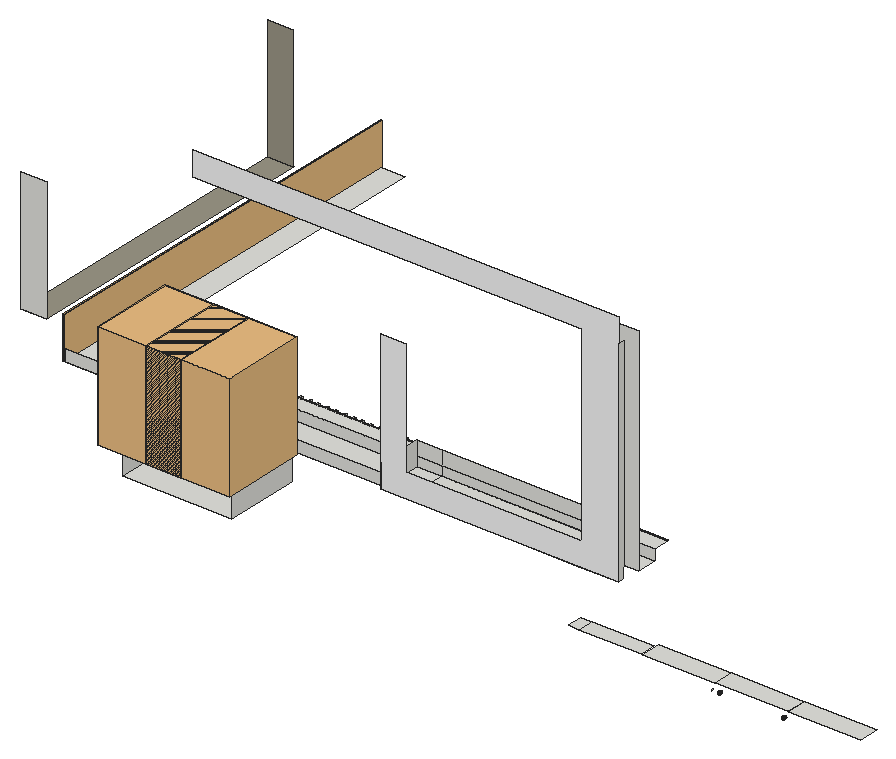
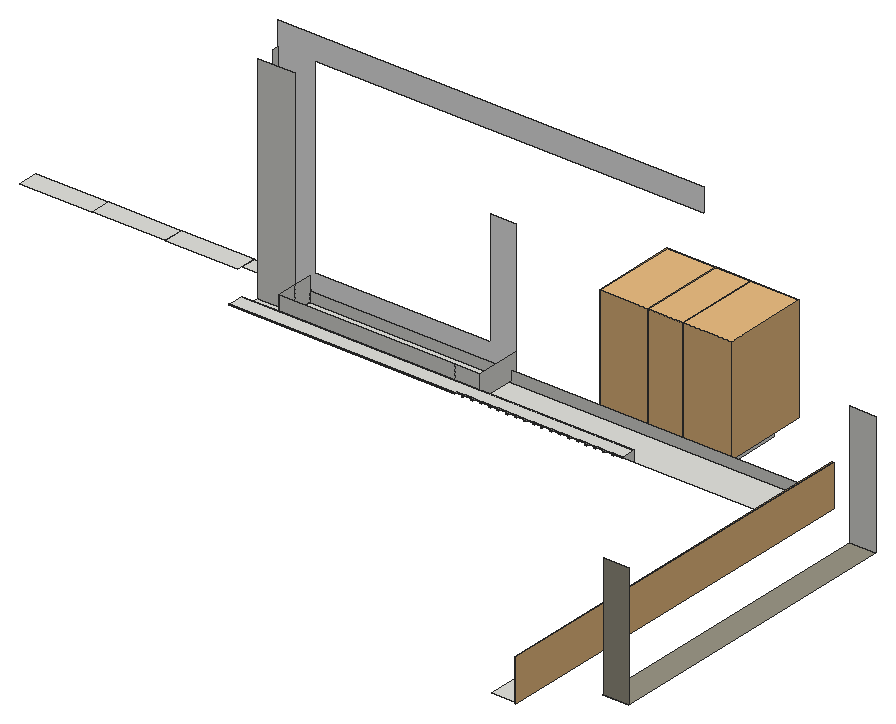
# SketchUp Ruby script. Lengths in inches.
U = 1.inch
M = Sketchup.active_model
def pt(a) = Geom::Point3d.new(a.map { |v| v * U })
def face(e, loops, mat)
  f = e.add_face(loops[0].map { |a| pt(a) })
  loops[1..].each { |l| e.add_face(l.map { |a| pt(a) }).erase! }
  f.material = f.back_material = mat if mat
  f
end
# faces: each face lists its corners as indices into pts; further lists are holes
def faces(e, pts, list, mat = nil) = list.each { |f| face(e, (f[0].is_a?(Array) ? f : [f]).map { |l| l.map { |i| pts[i] } }, mat) }
# xy, xz, yz: faces in a plane at the given z, y or x. An outline is a flat list of corners, or four numbers for a rectangle; further outlines are holes
def ring(l) = l.size == 4 ? [[l[0], l[1]], [l[2], l[1]], [l[2], l[3]], [l[0], l[3]]] : l.each_slice(2).to_a
def flat(e, list, mat, &to3) = list.each { |f| face(e, (f[0].is_a?(Array) ? f : [f]).map { |l| ring(l).map { |u, v| to3.(u, v) } }, mat) }
def xy(e, z, list, mat = nil) = flat(e, list, mat) { |x, y| [x, y, z] }
def xz(e, y, list, mat = nil) = flat(e, list, mat) { |x, z| [x, y, z] }
def yz(e, x, list, mat = nil) = flat(e, list, mat) { |y, z| [x, y, z] }
def lines(e, pts, list) = list.each { |a, b| e.add_line(pt(pts[a]), pt(pts[b])) }
# prism: a flat outline (further loops are holes) pulled along v
def prism(e, loops, v, mat = nil)
  f = face(e, loops, mat); d = Geom::Vector3d.new(v.map { |x| x * U })
  f.pushpull(f.normal.samedirection?(d) ? d.length : -d.length)
end
def box(e, o, s, mat = nil) = prism(e, [[o, [o[0] + s[0], o[1], o[2]], [o[0] + s[0], o[1] + s[1], o[2]], [o[0], o[1] + s[1], o[2]]]], [0, 0, s[2]], mat)
def at(x, y, z, deg = 0) = Geom::Transformation.translation(pt([x, y, z])) * Geom::Transformation.rotation(ORIGIN, Z_AXIS, deg.degrees)
def axes(o, x, y, z) = Geom::Transformation.new([*x, 0, *y, 0, *z, 0, *pt(o).to_a, 1])
def part(name) = M.definitions.add(name)
# library, detail: a bought-in or finely detailed component or shape, given as its bounding box
def library(name, o, s) = part(name).tap { |d| box(d.entities, o, s) }
def detail(e, o, s) = box(e.add_group.entities, o, s)
def put(e, d, t, mat = nil) = e.add_instance(d, t).tap { |i| i.material = mat if mat }
def group(e, t, mat = nil) = e.add_group.tap { |g| g.transformation = t; g.material = mat if mat }.entities
root = M.entities
M.materials.add("[0129_WhiteSmoke]1").color = [245, 245, 245]
M.materials.add("[Concrete Tile]").color = [155, 150, 134]
c1 = library("plant (1)",[-35.72,-28.42,0],[66.31,67.39,84.38])
c2 = part("glass-railing")
detail(c2.entities,[0,0,0],[1.26,75.59,33.1875])
xy(root,138.0625,[[3488.55,801.78,3496.96,814.22],[3496.96,801.78,3546.61,814.22],[3547.54,801.78,3604.66,817.6],[3605.72,801.78,3662.71,817.6],[3664.02,801.78,3720.76,817.6]])
xy(root,138.1875,[[3153.83,776.37,3240.72,836.7]])
xy(root,153.5625,[[3050.93,846.1,3467.75,846.1,3467.75,861.24,3496.96,861.24,3496.96,877.14,3071.34,877.14,3071.34,1160.85,3050.93,1160.85]])
xy(root,154.75,[[3307.68,840.97,3327.33,877.14],[3327.33,840.97,3467.75,877.14],[3467.75,840.97,3496.96,845.35]])
xy(root,156.5,[[2992.01,877.14,3012.76,1122.97]],"[Concrete Tile]")
xy(root,162.125,[[3184.99,877.14,3184.99,888.95,3190.41,888.95,3190.41,890.39,3192.05,890.39,3192.05,888.95,3197.47,888.95,3197.47,890.39,3199.05,890.39,3199.05,888.95,3204.47,888.95,3204.47,890.39,3206.05,890.39,3206.05,888.95,3211.47,888.95,3211.47,890.39,3213.05,890.39,3213.05,888.95,3218.47,888.95,3218.47,890.39,3220.05,890.39,3220.05,888.95,3225.47,888.95,3225.47,890.39,3227.05,890.39,3227.05,888.95,3232.47,888.95,3232.47,890.39,3234.05,890.39,3234.05,888.95,3239.47,888.95,3239.47,890.39,3241.05,890.39,3241.05,888.95,3246.47,888.95,3246.47,890.39,3248.05,890.39,3248.05,888.95,3253.47,888.95,3253.47,890.39,3255.05,890.39,3255.05,888.95,3260.47,888.95,3260.47,890.39,3262.05,890.39,3262.05,888.95,3267.47,888.95,3267.47,890.39,3269.05,890.39,3269.05,888.95,3274.47,888.95,3274.47,890.39,3276.05,890.39,3276.05,888.83,3281.47,888.83,3281.47,890.39,3283.05,890.39,3283.05,888.83,3288.47,888.83,3288.47,890.39,3290.05,890.39,3290.05,888.83,3295.47,888.83,3295.47,890.39,3297.05,890.39,3297.05,888.83,3302.47,888.83,3302.47,890.39,3304.05,890.39,3304.05,888.83,3309.47,888.83,3309.47,890.39,3311.05,890.39,3311.05,888.83,3316.47,888.83,3316.47,890.39,3496.96,890.39,3496.96,877.14]])
xz(root,836.7,[[3153.83,138.1875,3240.72,183.3125]])
xz(root,840.97,[[3307.68,154.75,3496.96,154.75,3496.96,343.4375,3158.3,343.4375,3158.3,324.5625,3467.75,324.5625,3467.75,173.4375,3327.33,173.4375,3327.33,264.75,3307.68,264.75]],"[0129_WhiteSmoke]1")
xz(root,845.35,[[3467.75,154.75,3496.96,163]])
xz(root,846.1,[[3050.93,153.5625,3467.75,162.75]])
xz(root,861.24,[[3467.75,153.5625,3496.96,324.5625]])
xz(root,877.14,[[3184.99,153.5625,3496.96,153.5625,3496.96,162.125,3467.75,162.125,3467.75,154.75,3307.68,154.75,3307.68,162.125,3184.99,162.125],[3307.68,154.75,3327.33,162.125],[3327.33,154.75,3467.75,162.125],[2992.01,156.5,3012.76,254.125],[3307.68,162.125,3327.33,173.4375],
  [3327.33,162.125,3467.75,173.4375]])
xz(root,888.83,[[3276.05,162.125,3281.47,162.75],[3283.05,162.125,3288.47,162.75],[3290.05,162.125,3295.47,162.75],[3297.05,162.125,3302.47,162.75],[3304.05,162.125,3309.47,162.75],
  [3311.05,162.125,3316.47,162.75]])
xz(root,888.95,[[3184.99,162.125,3190.41,162.75],[3192.05,162.125,3197.47,162.75],[3199.05,162.125,3204.47,162.75],[3206.05,162.125,3211.47,162.75],[3213.05,162.125,3218.47,162.75],
  [3220.05,162.125,3225.47,162.75],[3227.05,162.125,3232.47,162.75],[3234.05,162.125,3239.47,162.75],[3241.05,162.125,3246.47,162.75],[3248.05,162.125,3253.47,162.75],
  [3255.05,162.125,3260.47,162.75],[3262.05,162.125,3267.47,162.75],[3269.05,162.125,3274.47,162.75]])
xz(root,890.39,[[3190.41,162.125,3192.05,162.75],[3197.47,162.125,3199.05,162.75],[3204.47,162.125,3206.05,162.75],[3211.47,162.125,3213.05,162.75],[3218.47,162.125,3220.05,162.75],
  [3225.47,162.125,3227.05,162.75],[3232.47,162.125,3234.05,162.75],[3239.47,162.125,3241.05,162.75],[3246.47,162.125,3248.05,162.75],[3253.47,162.125,3255.05,162.75],
  [3260.47,162.125,3262.05,162.75],[3267.47,162.125,3269.05,162.75],[3274.47,162.125,3276.05,162.75],[3281.47,162.125,3283.05,162.75],[3288.47,162.125,3290.05,162.75],
  [3295.47,162.125,3297.05,162.75],[3302.47,162.125,3304.05,162.75],[3309.47,162.125,3311.05,162.75],[3316.47,162.125,3319.59,162.75],[3319.59,162.125,3496.96,162.75]])
xz(root,1122.97,[[2992.01,156.5,3012.13,254.125]],"[Concrete Tile]")
yz(root,3153.83,[[776.37,138.1875,836.7,183.3125]])
yz(root,3190.41,[[888.95,162.125,890.39,162.75]])
yz(root,3192.05,[[888.95,162.125,890.39,162.75]])
yz(root,3197.47,[[888.95,162.125,890.39,162.75]])
yz(root,3199.05,[[888.95,162.125,890.39,162.75]])
yz(root,3204.47,[[888.95,162.125,890.39,162.75]])
yz(root,3206.05,[[888.95,162.125,890.39,162.75]])
yz(root,3211.47,[[888.95,162.125,890.39,162.75]])
yz(root,3213.05,[[888.95,162.125,890.39,162.75]])
yz(root,3218.47,[[888.95,162.125,890.39,162.75]])
yz(root,3220.05,[[888.95,162.125,890.39,162.75]])
yz(root,3225.47,[[888.95,162.125,890.39,162.75]])
yz(root,3227.05,[[888.95,162.125,890.39,162.75]])
yz(root,3232.47,[[888.95,162.125,890.39,162.75]])
yz(root,3234.05,[[888.95,162.125,890.39,162.75]])
yz(root,3239.47,[[888.95,162.125,890.39,162.75]])
yz(root,3240.72,[[776.37,138.1875,836.7,183.3125]])
yz(root,3241.05,[[888.95,162.125,890.39,162.75]])
yz(root,3246.47,[[888.95,162.125,890.39,162.75]])
yz(root,3248.05,[[888.95,162.125,890.39,162.75]])
yz(root,3253.47,[[888.95,162.125,890.39,162.75]])
yz(root,3255.05,[[888.95,162.125,890.39,162.75]])
yz(root,3260.47,[[888.95,162.125,890.39,162.75]])
yz(root,3262.05,[[888.95,162.125,890.39,162.75]])
yz(root,3267.47,[[888.95,162.125,890.39,162.75]])
yz(root,3269.05,[[888.95,162.125,890.39,162.75]])
yz(root,3274.47,[[888.95,162.125,890.39,162.75]])
yz(root,3276.05,[[888.83,162.125,890.39,162.75]])
yz(root,3281.47,[[888.83,162.125,890.39,162.75]])
yz(root,3283.05,[[888.83,162.125,890.39,162.75]])
yz(root,3288.47,[[888.83,162.125,890.39,162.75]])
yz(root,3290.05,[[888.83,162.125,890.39,162.75]])
yz(root,3295.47,[[888.83,162.125,890.39,162.75]])
yz(root,3297.05,[[888.83,162.125,890.39,162.75]])
yz(root,3302.47,[[888.83,162.125,890.39,162.75]])
yz(root,3304.05,[[888.83,162.125,890.39,162.75]])
yz(root,3307.68,[[840.97,154.75,877.14,173.4375]])
yz(root,3309.47,[[888.83,162.125,890.39,162.75]])
yz(root,3311.05,[[888.83,162.125,890.39,162.75]])
yz(root,3316.47,[[888.83,162.125,890.39,162.75]])
yz(root,3467.75,[[846.1,153.5625,861.24,154.75],[845.35,154.75,846.1,162.75],[846.1,154.75,861.24,173.4375],[861.24,154.75,877.14,173.4375]])
yz(root,3496.96,[[840.97,154.75,845.35,154.75,845.35,163,846.1,163,846.1,324.5625,840.97,324.5625]])
p = [[3609.04,801.78,132.03],[3609.3125,801.78,131.92],[3609.3125,799.91,131.92],[3609.04,799.91,132.03],[3609.6,801.78,131.88],[3609.6,799.91,131.88],
  [3609.9,801.78,131.92],[3609.9,799.91,131.92],[3610.17,801.78,132.03],[3610.17,799.91,132.03],[3660.17,801.78,132.03],[3660.4375,801.78,131.92],
  [3660.4375,799.91,131.92],[3660.17,799.91,132.03],[3660.73,801.78,131.88],[3660.73,799.91,131.88],[3661.02,801.78,131.92],[3661.02,799.91,131.92],
  [3661.29,801.78,132.03],[3661.29,799.91,132.03],[3608.81,801.78,132.21],[3608.81,799.91,132.21],[3610.4,801.78,132.21],[3610.4,799.91,132.21],
  [3659.93,801.78,132.21],[3659.93,799.91,132.21],[3661.53,801.78,132.21],[3661.53,799.91,132.21],[3608.63,801.78,132.44],[3608.63,799.91,132.44],
  [3610.58,801.78,132.44],[3610.58,799.91,132.44],[3659.76,801.78,132.44],[3659.76,799.91,132.44],[3661.7,801.78,132.44],[3661.7,799.91,132.44],
  [3608.52,801.78,132.71],[3608.52,799.91,132.71],[3610.69,801.78,132.71],[3610.69,799.91,132.71],[3659.64,801.78,132.71],[3659.64,799.91,132.71],
  [3661.82,801.78,132.71],[3661.82,799.91,132.71],[3603.64,801.78,132.71],[3603.68,801.78,133],[3603.68,799.91,133],[3603.64,799.91,132.71],
  [3608.48,801.78,133],[3608.48,799.91,133],[3610.73,801.78,133],[3610.73,799.91,133],[3659.6,801.78,133],[3659.6,799.91,133],
  [3661.85,801.78,133],[3661.85,799.91,133],[3608.52,801.78,133.29],[3608.52,799.91,133.29],[3610.69,801.78,133.29],[3610.69,799.91,133.29],
  [3659.64,801.78,133.29],[3659.64,799.91,133.29],[3661.82,801.78,133.29],[3661.82,799.91,133.29],[3608.63,801.78,133.57],[3608.63,799.91,133.57],
  [3610.58,801.78,133.57],[3610.58,799.91,133.57],[3659.76,801.78,133.57],[3659.76,799.91,133.57],[3661.7,801.78,133.57],[3661.7,799.91,133.57],
  [3608.81,801.78,133.8],[3608.81,799.91,133.8],[3610.4,801.78,133.8],[3610.4,799.91,133.8],[3659.93,801.78,133.8],[3659.93,799.91,133.8],
  [3661.53,801.78,133.8],[3661.53,799.91,133.8],[3609.04,801.78,133.98],[3609.04,799.91,133.98],[3610.17,801.78,133.98],[3610.17,799.91,133.98],
  [3660.17,801.78,133.98],[3660.17,799.91,133.98],[3661.29,801.78,133.98],[3661.29,799.91,133.98],[3609.3125,801.78,134.09],[3609.3125,799.91,134.09],
  [3609.9,801.78,134.09],[3609.9,799.91,134.09],[3660.4375,801.78,134.09],[3660.4375,799.91,134.09],[3661.02,801.78,134.09],[3661.02,799.91,134.09],
  [3609.6,801.78,134.13],[3609.6,799.91,134.13],[3660.73,801.78,134.13],[3660.73,799.91,134.13]]
faces(root,p,[[0,1,2,3],[1,4,5,2],[4,6,7,5],[6,8,9,7],[10,11,12,13],[11,14,15,12],[14,16,17,15],[16,18,19,17],
  [20,0,3,21],[8,22,23,9],[24,10,13,25],[18,26,27,19],[28,20,21,29],[22,30,31,23],[32,24,25,33],[26,34,35,27],
  [36,28,29,37],[30,38,39,31],[40,32,33,41],[34,42,43,35],[44,45,46,47],[48,36,37,49],[38,50,51,39],[52,40,41,53],
  [42,54,55,43],[56,48,49,57],[50,58,59,51],[60,52,53,61],[54,62,63,55],[64,56,57,65],[58,66,67,59],[68,60,61,69],
  [62,70,71,63],[72,64,65,73],[66,74,75,67],[76,68,69,77],[70,78,79,71],[80,72,73,81],[74,82,83,75],[84,76,77,85],
  [78,86,87,79],[88,80,81,89],[82,90,91,83],[92,84,85,93],[86,94,95,87],[96,88,89,97],[90,96,97,91],[98,92,93,99],
  [94,98,99,95]])
put(root,c1,at(3172.85,800.97,155.86))
put(root,c1,at(3211.41,800.97,155.86))
put(root,c2,axes([3050.93,846.1,153.5625],[1,0,0],[0,4.1738,0],[0,0,1]))
